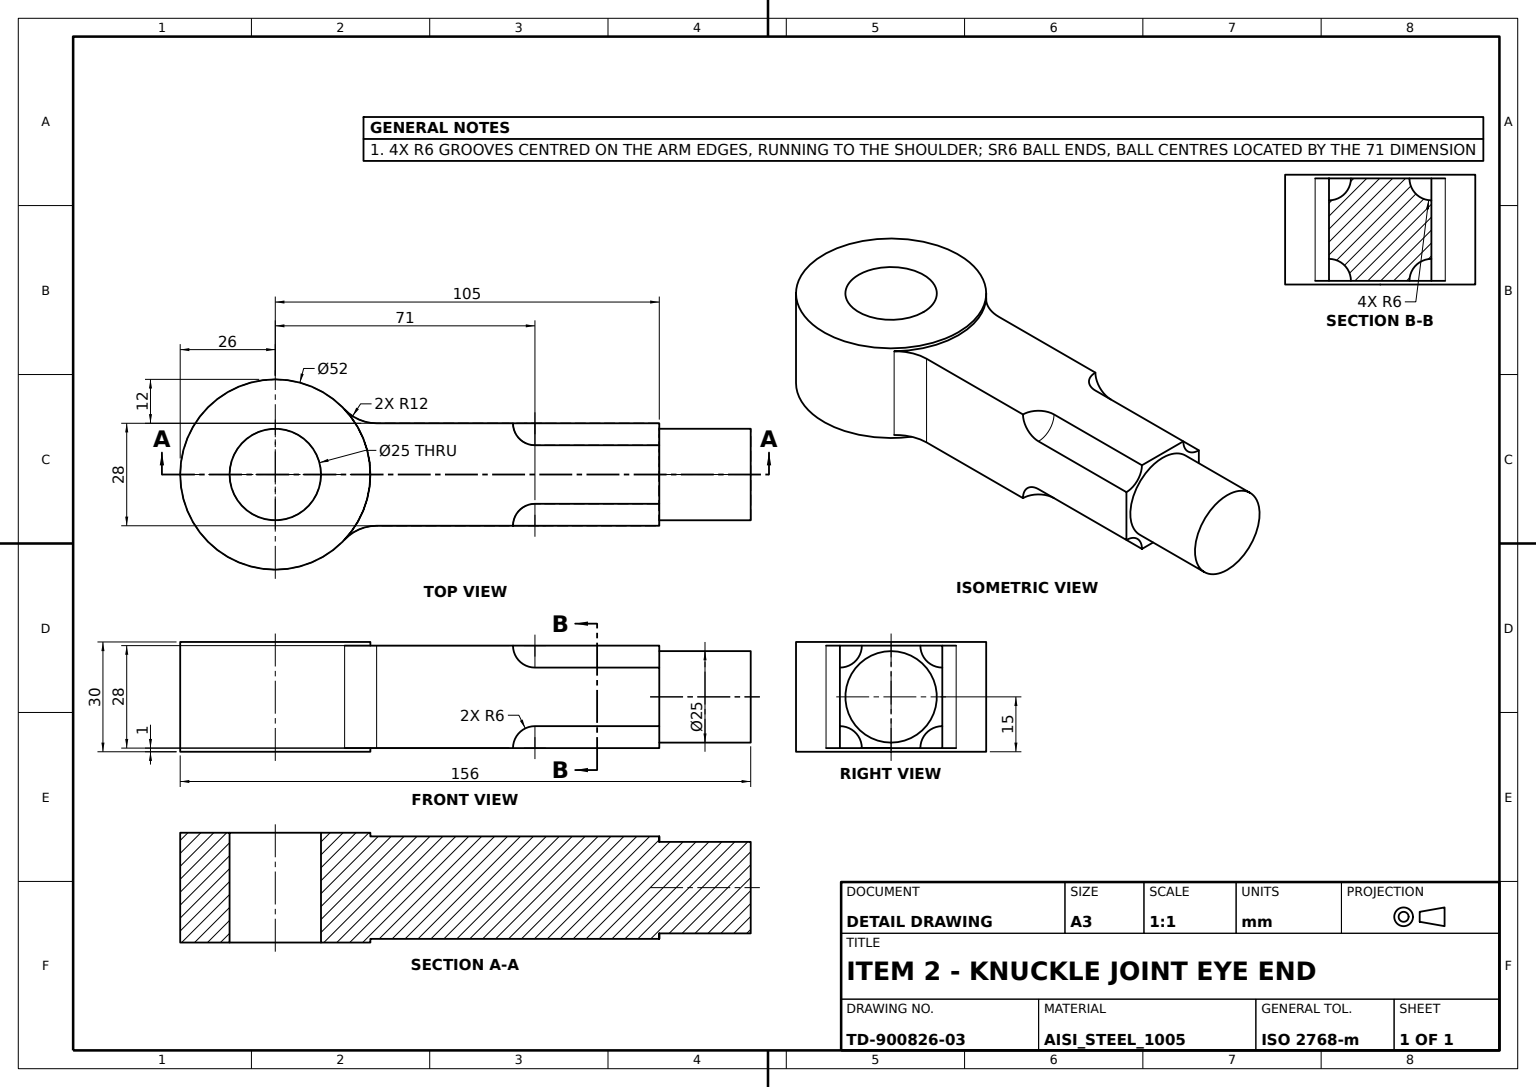
ISO-10303-21;
HEADER;
FILE_DESCRIPTION((''),'2;1');
FILE_NAME('','',(''),(''),'','','');
FILE_SCHEMA(('AUTOMOTIVE_DESIGN'));
ENDSEC;
DATA;
#1=APPLICATION_CONTEXT('');
#2=PRODUCT_CONTEXT('',#1,'mechanical');
#3=PRODUCT('','','',(#2));
#4=PRODUCT_DEFINITION_FORMATION('','',#3);
#5=PRODUCT_DEFINITION_CONTEXT('',#1,'design');
#6=PRODUCT_DEFINITION('','',#4,#5);
#7=PRODUCT_DEFINITION_SHAPE('','',#6);
#8=(LENGTH_UNIT()NAMED_UNIT(*)SI_UNIT(.MILLI.,.METRE.));
#9=(NAMED_UNIT(*)PLANE_ANGLE_UNIT()SI_UNIT($,.RADIAN.));
#10=(NAMED_UNIT(*)SI_UNIT($,.STERADIAN.)SOLID_ANGLE_UNIT());
#11=UNCERTAINTY_MEASURE_WITH_UNIT(LENGTH_MEASURE(0.005),#8,'distance_accuracy_value','');
#12=(GEOMETRIC_REPRESENTATION_CONTEXT(3)GLOBAL_UNCERTAINTY_ASSIGNED_CONTEXT((#11))GLOBAL_UNIT_ASSIGNED_CONTEXT((#8,#9,#10))REPRESENTATION_CONTEXT('',''));
#13=CARTESIAN_POINT('',(105.,-14.,-8.));
#14=VERTEX_POINT('',#13);
#15=CARTESIAN_POINT('',(105.,-8.,-14.));
#16=VERTEX_POINT('',#15);
#17=CARTESIAN_POINT('',(105.,-14.,-14.));
#18=DIRECTION('',(-1.,0.,0.));
#19=DIRECTION('',(0.,1.,0.));
#20=AXIS2_PLACEMENT_3D('',#17,#18,#19);
#21=CIRCLE('',#20,6.);
#22=EDGE_CURVE('',#14,#16,#21,.T.);
#23=ORIENTED_EDGE('',*,*,#22,.F.);
#24=CARTESIAN_POINT('',(71.,-14.,-8.));
#25=VERTEX_POINT('',#24);
#26=CARTESIAN_POINT('',(65.,-14.,-8.));
#27=DIRECTION('',(1.,0.,0.));
#28=VECTOR('',#27,1000.);
#29=LINE('',#26,#28);
#30=EDGE_CURVE('',#25,#14,#29,.T.);
#31=ORIENTED_EDGE('',*,*,#30,.F.);
#32=CARTESIAN_POINT('',(71.,-8.,-14.));
#33=VERTEX_POINT('',#32);
#34=CARTESIAN_POINT('',(71.,-14.,-14.));
#35=DIRECTION('',(0.,0.,-1.));
#36=AXIS2_PLACEMENT_3D('',#34,#27,#35);
#37=CIRCLE('',#36,6.);
#38=EDGE_CURVE('',#25,#33,#37,.F.);
#39=ORIENTED_EDGE('',*,*,#38,.T.);
#40=CARTESIAN_POINT('',(65.,-8.,-14.));
#41=LINE('',#40,#28);
#42=EDGE_CURVE('',#33,#16,#41,.T.);
#43=ORIENTED_EDGE('',*,*,#42,.T.);
#44=EDGE_LOOP('',(#23,#31,#39,#43));
#45=FACE_BOUND('',#44,.T.);
#46=CARTESIAN_POINT('',(65.,-14.,-14.));
#47=AXIS2_PLACEMENT_3D('',#46,#27,#35);
#48=CYLINDRICAL_SURFACE('',#47,6.);
#49=ADVANCED_FACE('',(#45),#48,.F.);
#50=ORIENTED_EDGE('',*,*,#42,.F.);
#51=VERTEX_POINT('',#46);
#52=DIRECTION('',(0.,0.,1.));
#53=AXIS2_PLACEMENT_3D('',#34,#52,#27);
#54=CIRCLE('',#53,6.);
#55=EDGE_CURVE('',#33,#51,#54,.T.);
#56=ORIENTED_EDGE('',*,*,#55,.T.);
#57=CARTESIAN_POINT('',(27.712813,-14.,-14.));
#58=VERTEX_POINT('',#57);
#59=VECTOR('',#18,1000.);
#60=LINE('',#17,#59);
#61=EDGE_CURVE('',#51,#58,#60,.T.);
#62=ORIENTED_EDGE('',*,*,#61,.T.);
#63=CARTESIAN_POINT('',(18.961398,-17.789474,-14.));
#64=VERTEX_POINT('',#63);
#65=CARTESIAN_POINT('',(27.712813,-26.,-14.));
#66=AXIS2_PLACEMENT_3D('',#65,#52,#27);
#67=CIRCLE('',#66,12.);
#68=EDGE_CURVE('',#58,#64,#67,.T.);
#69=ORIENTED_EDGE('',*,*,#68,.T.);
#70=CARTESIAN_POINT('',(18.961398,17.789474,-14.));
#71=VERTEX_POINT('',#70);
#72=CARTESIAN_POINT('',(0.,0.,-14.));
#73=AXIS2_PLACEMENT_3D('',#72,#52,#27);
#74=CIRCLE('',#73,26.);
#75=EDGE_CURVE('',#64,#71,#74,.T.);
#76=ORIENTED_EDGE('',*,*,#75,.T.);
#77=CARTESIAN_POINT('',(27.712813,14.,-14.));
#78=VERTEX_POINT('',#77);
#79=CARTESIAN_POINT('',(27.712813,26.,-14.));
#80=AXIS2_PLACEMENT_3D('',#79,#52,#27);
#81=CIRCLE('',#80,12.);
#82=EDGE_CURVE('',#71,#78,#81,.T.);
#83=ORIENTED_EDGE('',*,*,#82,.T.);
#84=CARTESIAN_POINT('',(65.,14.,-14.));
#85=VERTEX_POINT('',#84);
#86=CARTESIAN_POINT('',(21.908902,14.,-14.));
#87=LINE('',#86,#28);
#88=EDGE_CURVE('',#78,#85,#87,.T.);
#89=ORIENTED_EDGE('',*,*,#88,.T.);
#90=CARTESIAN_POINT('',(71.,8.,-14.));
#91=VERTEX_POINT('',#90);
#92=CARTESIAN_POINT('',(71.,14.,-14.));
#93=AXIS2_PLACEMENT_3D('',#92,#52,#27);
#94=CIRCLE('',#93,6.);
#95=EDGE_CURVE('',#85,#91,#94,.T.);
#96=ORIENTED_EDGE('',*,*,#95,.T.);
#97=CARTESIAN_POINT('',(105.,8.,-14.));
#98=VERTEX_POINT('',#97);
#99=CARTESIAN_POINT('',(65.,8.,-14.));
#100=LINE('',#99,#28);
#101=EDGE_CURVE('',#91,#98,#100,.T.);
#102=ORIENTED_EDGE('',*,*,#101,.T.);
#103=CARTESIAN_POINT('',(105.,14.,-14.));
#104=DIRECTION('',(0.,-1.,0.));
#105=VECTOR('',#104,1000.);
#106=LINE('',#103,#105);
#107=EDGE_CURVE('',#98,#16,#106,.T.);
#108=ORIENTED_EDGE('',*,*,#107,.T.);
#109=EDGE_LOOP('',(#50,#56,#62,#69,#76,#83,#89,#96,#102,#108));
#110=FACE_BOUND('',#109,.T.);
#111=PLANE('',#73);
#112=ADVANCED_FACE('',(#110),#111,.F.);
#113=CARTESIAN_POINT('',(71.,14.,-8.));
#114=VERTEX_POINT('',#113);
#115=AXIS2_PLACEMENT_3D('',#92,#19,#52);
#116=CIRCLE('',#115,6.);
#117=EDGE_CURVE('',#114,#85,#116,.F.);
#118=ORIENTED_EDGE('',*,*,#117,.F.);
#119=AXIS2_PLACEMENT_3D('',#92,#27,#35);
#120=CIRCLE('',#119,6.);
#121=EDGE_CURVE('',#91,#114,#120,.F.);
#122=ORIENTED_EDGE('',*,*,#121,.F.);
#123=ORIENTED_EDGE('',*,*,#95,.F.);
#124=EDGE_LOOP('',(#118,#122,#123));
#125=FACE_BOUND('',#124,.T.);
#126=AXIS2_PLACEMENT_3D('',#92,#18,#52);
#127=SPHERICAL_SURFACE('',#126,6.);
#128=ADVANCED_FACE('',(#125),#127,.F.);
#129=CARTESIAN_POINT('',(27.712813,14.,14.));
#130=VERTEX_POINT('',#129);
#131=CARTESIAN_POINT('',(18.961398,17.789474,14.));
#132=VERTEX_POINT('',#131);
#133=CARTESIAN_POINT('',(27.712813,26.,14.));
#134=AXIS2_PLACEMENT_3D('',#133,#52,#27);
#135=CIRCLE('',#134,12.);
#136=EDGE_CURVE('',#130,#132,#135,.F.);
#137=ORIENTED_EDGE('',*,*,#136,.F.);
#138=VECTOR('',#35,1000.);
#139=LINE('',#129,#138);
#140=EDGE_CURVE('',#78,#130,#139,.F.);
#141=ORIENTED_EDGE('',*,*,#140,.F.);
#142=ORIENTED_EDGE('',*,*,#82,.F.);
#143=CARTESIAN_POINT('',(18.961398,17.789474,15.));
#144=LINE('',#143,#138);
#145=EDGE_CURVE('',#132,#71,#144,.T.);
#146=ORIENTED_EDGE('',*,*,#145,.F.);
#147=EDGE_LOOP('',(#137,#141,#142,#146));
#148=FACE_BOUND('',#147,.T.);
#149=CARTESIAN_POINT('',(27.712813,26.,15.));
#150=AXIS2_PLACEMENT_3D('',#149,#35,#18);
#151=CYLINDRICAL_SURFACE('',#150,12.);
#152=ADVANCED_FACE('',(#148),#151,.F.);
#153=ORIENTED_EDGE('',*,*,#38,.F.);
#154=AXIS2_PLACEMENT_3D('',#34,#104,#35);
#155=CIRCLE('',#154,6.);
#156=EDGE_CURVE('',#51,#25,#155,.F.);
#157=ORIENTED_EDGE('',*,*,#156,.F.);
#158=ORIENTED_EDGE('',*,*,#55,.F.);
#159=EDGE_LOOP('',(#153,#157,#158));
#160=FACE_BOUND('',#159,.T.);
#161=AXIS2_PLACEMENT_3D('',#34,#18,#52);
#162=SPHERICAL_SURFACE('',#161,6.);
#163=ADVANCED_FACE('',(#160),#162,.F.);
#164=CARTESIAN_POINT('',(71.,8.,14.));
#165=VERTEX_POINT('',#164);
#166=CARTESIAN_POINT('',(65.,14.,14.));
#167=VERTEX_POINT('',#166);
#168=CARTESIAN_POINT('',(71.,14.,14.));
#169=AXIS2_PLACEMENT_3D('',#168,#52,#27);
#170=CIRCLE('',#169,6.);
#171=EDGE_CURVE('',#165,#167,#170,.F.);
#172=ORIENTED_EDGE('',*,*,#171,.F.);
#173=CARTESIAN_POINT('',(71.,14.,8.));
#174=VERTEX_POINT('',#173);
#175=AXIS2_PLACEMENT_3D('',#168,#27,#35);
#176=CIRCLE('',#175,6.);
#177=EDGE_CURVE('',#174,#165,#176,.F.);
#178=ORIENTED_EDGE('',*,*,#177,.F.);
#179=AXIS2_PLACEMENT_3D('',#168,#19,#52);
#180=CIRCLE('',#179,6.);
#181=EDGE_CURVE('',#167,#174,#180,.F.);
#182=ORIENTED_EDGE('',*,*,#181,.F.);
#183=EDGE_LOOP('',(#172,#178,#182));
#184=FACE_BOUND('',#183,.T.);
#185=SPHERICAL_SURFACE('',#175,6.);
#186=ADVANCED_FACE('',(#184),#185,.F.);
#187=CARTESIAN_POINT('',(105.,0.,-12.5));
#188=VERTEX_POINT('',#187);
#189=CARTESIAN_POINT('',(105.,0.,0.));
#190=AXIS2_PLACEMENT_3D('',#189,#27,#35);
#191=CIRCLE('',#190,12.5);
#192=EDGE_CURVE('',#188,#188,#191,.T.);
#193=ORIENTED_EDGE('',*,*,#192,.F.);
#194=EDGE_LOOP('',(#193));
#195=FACE_BOUND('',#194,.T.);
#196=CARTESIAN_POINT('',(105.,14.,8.));
#197=VERTEX_POINT('',#196);
#198=CARTESIAN_POINT('',(105.,14.,-8.));
#199=VERTEX_POINT('',#198);
#200=CARTESIAN_POINT('',(105.,14.,14.));
#201=LINE('',#200,#138);
#202=EDGE_CURVE('',#197,#199,#201,.T.);
#203=ORIENTED_EDGE('',*,*,#202,.F.);
#204=CARTESIAN_POINT('',(105.,8.,14.));
#205=VERTEX_POINT('',#204);
#206=AXIS2_PLACEMENT_3D('',#200,#27,#19);
#207=CIRCLE('',#206,6.);
#208=EDGE_CURVE('',#205,#197,#207,.T.);
#209=ORIENTED_EDGE('',*,*,#208,.F.);
#210=CARTESIAN_POINT('',(105.,-8.,14.));
#211=VERTEX_POINT('',#210);
#212=LINE('',#200,#105);
#213=EDGE_CURVE('',#205,#211,#212,.T.);
#214=ORIENTED_EDGE('',*,*,#213,.T.);
#215=CARTESIAN_POINT('',(105.,-14.,8.));
#216=VERTEX_POINT('',#215);
#217=CARTESIAN_POINT('',(105.,-14.,14.));
#218=AXIS2_PLACEMENT_3D('',#217,#18,#19);
#219=CIRCLE('',#218,6.);
#220=EDGE_CURVE('',#211,#216,#219,.T.);
#221=ORIENTED_EDGE('',*,*,#220,.T.);
#222=LINE('',#217,#138);
#223=EDGE_CURVE('',#216,#14,#222,.T.);
#224=ORIENTED_EDGE('',*,*,#223,.T.);
#225=ORIENTED_EDGE('',*,*,#22,.T.);
#226=ORIENTED_EDGE('',*,*,#107,.F.);
#227=AXIS2_PLACEMENT_3D('',#103,#18,#19);
#228=CIRCLE('',#227,6.);
#229=EDGE_CURVE('',#98,#199,#228,.T.);
#230=ORIENTED_EDGE('',*,*,#229,.T.);
#231=EDGE_LOOP('',(#203,#209,#214,#221,#224,#225,#226,#230));
#232=FACE_BOUND('',#231,.T.);
#233=AXIS2_PLACEMENT_3D('',#200,#27,#35);
#234=PLANE('',#233);
#235=ADVANCED_FACE('',(#195,#232),#234,.T.);
#236=CARTESIAN_POINT('',(18.961398,-17.789474,14.));
#237=VERTEX_POINT('',#236);
#238=CARTESIAN_POINT('',(27.712813,-14.,14.));
#239=VERTEX_POINT('',#238);
#240=CARTESIAN_POINT('',(27.712813,-26.,14.));
#241=AXIS2_PLACEMENT_3D('',#240,#52,#27);
#242=CIRCLE('',#241,12.);
#243=EDGE_CURVE('',#237,#239,#242,.F.);
#244=ORIENTED_EDGE('',*,*,#243,.F.);
#245=CARTESIAN_POINT('',(18.961398,-17.789474,15.));
#246=LINE('',#245,#138);
#247=EDGE_CURVE('',#64,#237,#246,.F.);
#248=ORIENTED_EDGE('',*,*,#247,.F.);
#249=ORIENTED_EDGE('',*,*,#68,.F.);
#250=LINE('',#238,#138);
#251=EDGE_CURVE('',#239,#58,#250,.T.);
#252=ORIENTED_EDGE('',*,*,#251,.F.);
#253=EDGE_LOOP('',(#244,#248,#249,#252));
#254=FACE_BOUND('',#253,.T.);
#255=CARTESIAN_POINT('',(27.712813,-26.,15.));
#256=AXIS2_PLACEMENT_3D('',#255,#35,#18);
#257=CYLINDRICAL_SURFACE('',#256,12.);
#258=ADVANCED_FACE('',(#254),#257,.F.);
#259=CARTESIAN_POINT('',(26.,0.,15.));
#260=VERTEX_POINT('',#259);
#261=CARTESIAN_POINT('',(0.,0.,15.));
#262=AXIS2_PLACEMENT_3D('',#261,#52,#27);
#263=CIRCLE('',#262,26.);
#264=EDGE_CURVE('',#260,#260,#263,.T.);
#265=ORIENTED_EDGE('',*,*,#264,.T.);
#266=EDGE_LOOP('',(#265));
#267=FACE_BOUND('',#266,.T.);
#268=CARTESIAN_POINT('',(12.5,0.,15.));
#269=VERTEX_POINT('',#268);
#270=AXIS2_PLACEMENT_3D('',#261,#35,#27);
#271=CIRCLE('',#270,12.5);
#272=EDGE_CURVE('',#269,#269,#271,.T.);
#273=ORIENTED_EDGE('',*,*,#272,.T.);
#274=EDGE_LOOP('',(#273));
#275=FACE_BOUND('',#274,.T.);
#276=PLANE('',#262);
#277=ADVANCED_FACE('',(#267,#275),#276,.T.);
#278=CARTESIAN_POINT('',(71.,-14.,8.));
#279=VERTEX_POINT('',#278);
#280=CARTESIAN_POINT('',(65.,-14.,8.));
#281=LINE('',#280,#28);
#282=EDGE_CURVE('',#279,#216,#281,.T.);
#283=ORIENTED_EDGE('',*,*,#282,.F.);
#284=CARTESIAN_POINT('',(65.,-14.,14.));
#285=VERTEX_POINT('',#284);
#286=CARTESIAN_POINT('',(71.,-14.,14.));
#287=AXIS2_PLACEMENT_3D('',#286,#104,#35);
#288=CIRCLE('',#287,6.);
#289=EDGE_CURVE('',#279,#285,#288,.F.);
#290=ORIENTED_EDGE('',*,*,#289,.T.);
#291=LINE('',#217,#59);
#292=EDGE_CURVE('',#285,#239,#291,.T.);
#293=ORIENTED_EDGE('',*,*,#292,.T.);
#294=ORIENTED_EDGE('',*,*,#251,.T.);
#295=ORIENTED_EDGE('',*,*,#61,.F.);
#296=ORIENTED_EDGE('',*,*,#156,.T.);
#297=ORIENTED_EDGE('',*,*,#30,.T.);
#298=ORIENTED_EDGE('',*,*,#223,.F.);
#299=EDGE_LOOP('',(#283,#290,#293,#294,#295,#296,#297,#298));
#300=FACE_BOUND('',#299,.T.);
#301=AXIS2_PLACEMENT_3D('',#217,#104,#35);
#302=PLANE('',#301);
#303=ADVANCED_FACE('',(#300),#302,.T.);
#304=CARTESIAN_POINT('',(65.,14.,8.));
#305=LINE('',#304,#28);
#306=EDGE_CURVE('',#174,#197,#305,.T.);
#307=ORIENTED_EDGE('',*,*,#306,.F.);
#308=ORIENTED_EDGE('',*,*,#177,.T.);
#309=CARTESIAN_POINT('',(65.,8.,14.));
#310=LINE('',#309,#28);
#311=EDGE_CURVE('',#165,#205,#310,.T.);
#312=ORIENTED_EDGE('',*,*,#311,.T.);
#313=ORIENTED_EDGE('',*,*,#208,.T.);
#314=EDGE_LOOP('',(#307,#308,#312,#313));
#315=FACE_BOUND('',#314,.T.);
#316=AXIS2_PLACEMENT_3D('',#166,#27,#35);
#317=CYLINDRICAL_SURFACE('',#316,6.);
#318=ADVANCED_FACE('',(#315),#317,.F.);
#319=ORIENTED_EDGE('',*,*,#282,.T.);
#320=ORIENTED_EDGE('',*,*,#220,.F.);
#321=CARTESIAN_POINT('',(71.,-8.,14.));
#322=VERTEX_POINT('',#321);
#323=CARTESIAN_POINT('',(65.,-8.,14.));
#324=LINE('',#323,#28);
#325=EDGE_CURVE('',#322,#211,#324,.T.);
#326=ORIENTED_EDGE('',*,*,#325,.F.);
#327=AXIS2_PLACEMENT_3D('',#286,#27,#35);
#328=CIRCLE('',#327,6.);
#329=EDGE_CURVE('',#322,#279,#328,.F.);
#330=ORIENTED_EDGE('',*,*,#329,.T.);
#331=EDGE_LOOP('',(#319,#320,#326,#330));
#332=FACE_BOUND('',#331,.T.);
#333=AXIS2_PLACEMENT_3D('',#284,#27,#35);
#334=CYLINDRICAL_SURFACE('',#333,6.);
#335=ADVANCED_FACE('',(#332),#334,.F.);
#336=ORIENTED_EDGE('',*,*,#311,.F.);
#337=ORIENTED_EDGE('',*,*,#171,.T.);
#338=CARTESIAN_POINT('',(21.908902,14.,14.));
#339=LINE('',#338,#28);
#340=EDGE_CURVE('',#130,#167,#339,.T.);
#341=ORIENTED_EDGE('',*,*,#340,.F.);
#342=ORIENTED_EDGE('',*,*,#136,.T.);
#343=CARTESIAN_POINT('',(0.,0.,14.));
#344=AXIS2_PLACEMENT_3D('',#343,#52,#27);
#345=CIRCLE('',#344,26.);
#346=EDGE_CURVE('',#237,#132,#345,.T.);
#347=ORIENTED_EDGE('',*,*,#346,.F.);
#348=ORIENTED_EDGE('',*,*,#243,.T.);
#349=ORIENTED_EDGE('',*,*,#292,.F.);
#350=AXIS2_PLACEMENT_3D('',#286,#52,#27);
#351=CIRCLE('',#350,6.);
#352=EDGE_CURVE('',#285,#322,#351,.F.);
#353=ORIENTED_EDGE('',*,*,#352,.T.);
#354=ORIENTED_EDGE('',*,*,#325,.T.);
#355=ORIENTED_EDGE('',*,*,#213,.F.);
#356=EDGE_LOOP('',(#336,#337,#341,#342,#347,#348,#349,#353,#354,#355));
#357=FACE_BOUND('',#356,.T.);
#358=PLANE('',#344);
#359=ADVANCED_FACE('',(#357),#358,.T.);
#360=ORIENTED_EDGE('',*,*,#272,.F.);
#361=EDGE_LOOP('',(#360));
#362=FACE_BOUND('',#361,.T.);
#363=CARTESIAN_POINT('',(12.5,0.,-15.));
#364=VERTEX_POINT('',#363);
#365=CARTESIAN_POINT('',(0.,0.,-15.));
#366=AXIS2_PLACEMENT_3D('',#365,#35,#27);
#367=CIRCLE('',#366,12.5);
#368=EDGE_CURVE('',#364,#364,#367,.T.);
#369=ORIENTED_EDGE('',*,*,#368,.T.);
#370=EDGE_LOOP('',(#369));
#371=FACE_BOUND('',#370,.T.);
#372=AXIS2_PLACEMENT_3D('',#261,#35,#18);
#373=CYLINDRICAL_SURFACE('',#372,12.5);
#374=ADVANCED_FACE('',(#362,#371),#373,.F.);
#375=ORIENTED_EDGE('',*,*,#329,.F.);
#376=ORIENTED_EDGE('',*,*,#352,.F.);
#377=ORIENTED_EDGE('',*,*,#289,.F.);
#378=EDGE_LOOP('',(#375,#376,#377));
#379=FACE_BOUND('',#378,.T.);
#380=AXIS2_PLACEMENT_3D('',#286,#18,#52);
#381=SPHERICAL_SURFACE('',#380,6.);
#382=ADVANCED_FACE('',(#379),#381,.F.);
#383=CARTESIAN_POINT('',(26.,0.,-15.));
#384=VERTEX_POINT('',#383);
#385=AXIS2_PLACEMENT_3D('',#365,#52,#27);
#386=CIRCLE('',#385,26.);
#387=EDGE_CURVE('',#384,#384,#386,.T.);
#388=ORIENTED_EDGE('',*,*,#387,.F.);
#389=EDGE_LOOP('',(#388));
#390=FACE_BOUND('',#389,.T.);
#391=ORIENTED_EDGE('',*,*,#368,.F.);
#392=EDGE_LOOP('',(#391));
#393=FACE_BOUND('',#392,.T.);
#394=PLANE('',#385);
#395=ADVANCED_FACE('',(#390,#393),#394,.F.);
#396=CARTESIAN_POINT('',(130.,0.,-12.5));
#397=VERTEX_POINT('',#396);
#398=CARTESIAN_POINT('',(130.,0.,0.));
#399=AXIS2_PLACEMENT_3D('',#398,#27,#35);
#400=CIRCLE('',#399,12.5);
#401=EDGE_CURVE('',#397,#397,#400,.T.);
#402=ORIENTED_EDGE('',*,*,#401,.T.);
#403=EDGE_LOOP('',(#402));
#404=FACE_BOUND('',#403,.T.);
#405=PLANE('',#399);
#406=ADVANCED_FACE('',(#404),#405,.T.);
#407=ORIENTED_EDGE('',*,*,#181,.T.);
#408=ORIENTED_EDGE('',*,*,#306,.T.);
#409=ORIENTED_EDGE('',*,*,#202,.T.);
#410=CARTESIAN_POINT('',(65.,14.,-8.));
#411=LINE('',#410,#28);
#412=EDGE_CURVE('',#114,#199,#411,.T.);
#413=ORIENTED_EDGE('',*,*,#412,.F.);
#414=ORIENTED_EDGE('',*,*,#117,.T.);
#415=ORIENTED_EDGE('',*,*,#88,.F.);
#416=ORIENTED_EDGE('',*,*,#140,.T.);
#417=ORIENTED_EDGE('',*,*,#340,.T.);
#418=EDGE_LOOP('',(#407,#408,#409,#413,#414,#415,#416,#417));
#419=FACE_BOUND('',#418,.T.);
#420=AXIS2_PLACEMENT_3D('',#338,#19,#52);
#421=PLANE('',#420);
#422=ADVANCED_FACE('',(#419),#421,.T.);
#423=ORIENTED_EDGE('',*,*,#387,.T.);
#424=EDGE_LOOP('',(#423));
#425=FACE_BOUND('',#424,.T.);
#426=ORIENTED_EDGE('',*,*,#264,.F.);
#427=EDGE_LOOP('',(#426));
#428=FACE_BOUND('',#427,.T.);
#429=ORIENTED_EDGE('',*,*,#145,.T.);
#430=ORIENTED_EDGE('',*,*,#75,.F.);
#431=ORIENTED_EDGE('',*,*,#247,.T.);
#432=ORIENTED_EDGE('',*,*,#346,.T.);
#433=EDGE_LOOP('',(#429,#430,#431,#432));
#434=FACE_BOUND('',#433,.T.);
#435=CYLINDRICAL_SURFACE('',#372,26.);
#436=ADVANCED_FACE('',(#425,#428,#434),#435,.T.);
#437=ORIENTED_EDGE('',*,*,#101,.F.);
#438=ORIENTED_EDGE('',*,*,#121,.T.);
#439=ORIENTED_EDGE('',*,*,#412,.T.);
#440=ORIENTED_EDGE('',*,*,#229,.F.);
#441=EDGE_LOOP('',(#437,#438,#439,#440));
#442=FACE_BOUND('',#441,.T.);
#443=AXIS2_PLACEMENT_3D('',#84,#27,#35);
#444=CYLINDRICAL_SURFACE('',#443,6.);
#445=ADVANCED_FACE('',(#442),#444,.F.);
#446=ORIENTED_EDGE('',*,*,#192,.T.);
#447=EDGE_LOOP('',(#446));
#448=FACE_BOUND('',#447,.T.);
#449=ORIENTED_EDGE('',*,*,#401,.F.);
#450=EDGE_LOOP('',(#449));
#451=FACE_BOUND('',#450,.T.);
#452=AXIS2_PLACEMENT_3D('',#398,#18,#52);
#453=CYLINDRICAL_SURFACE('',#452,12.5);
#454=ADVANCED_FACE('',(#448,#451),#453,.T.);
#455=CLOSED_SHELL('',(#49,#112,#128,#152,#163,#186,#235,#258,#277,#303,#318,#335,#359,#374,#382,#395,#406,#422,#436,#445,#454));
#456=MANIFOLD_SOLID_BREP('',#455);
#457=ADVANCED_BREP_SHAPE_REPRESENTATION('',(#456),#12);
#458=SHAPE_DEFINITION_REPRESENTATION(#7,#457);
ENDSEC;
END-ISO-10303-21;
